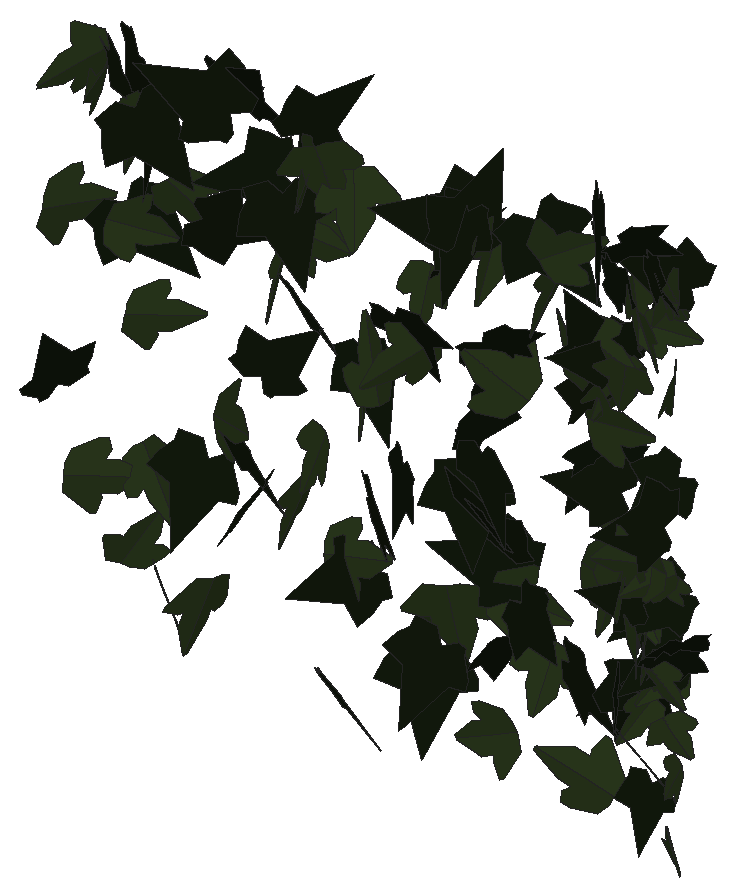
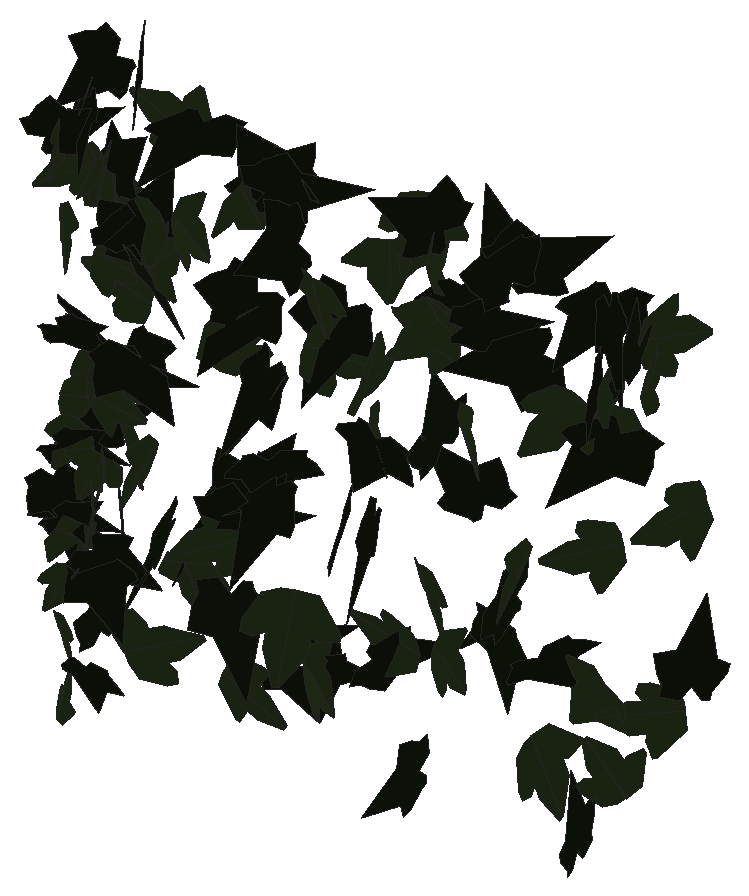
# SketchUp Ruby script. Lengths in inches.
U = 1.inch
M = Sketchup.active_model
def pt(a) = Geom::Point3d.new(a.map { |v| v * U })
def face(e, loops, mat)
  f = e.add_face(loops[0].map { |a| pt(a) })
  loops[1..].each { |l| e.add_face(l.map { |a| pt(a) }).erase! }
  f.material = f.back_material = mat if mat
  f
end
# faces: each face lists its corners as indices into pts; further lists are holes
def faces(e, pts, list, mat = nil) = list.each { |f| face(e, (f[0].is_a?(Array) ? f : [f]).map { |l| l.map { |i| pts[i] } }, mat) }
# xy, xz, yz: faces in a plane at the given z, y or x. An outline is a flat list of corners, or four numbers for a rectangle; further outlines are holes
def ring(l) = l.size == 4 ? [[l[0], l[1]], [l[2], l[1]], [l[2], l[3]], [l[0], l[3]]] : l.each_slice(2).to_a
def flat(e, list, mat, &to3) = list.each { |f| face(e, (f[0].is_a?(Array) ? f : [f]).map { |l| ring(l).map { |u, v| to3.(u, v) } }, mat) }
def xy(e, z, list, mat = nil) = flat(e, list, mat) { |x, y| [x, y, z] }
def xz(e, y, list, mat = nil) = flat(e, list, mat) { |x, z| [x, y, z] }
def yz(e, x, list, mat = nil) = flat(e, list, mat) { |y, z| [x, y, z] }
def lines(e, pts, list) = list.each { |a, b| e.add_line(pt(pts[a]), pt(pts[b])) }
# prism: a flat outline (further loops are holes) pulled along v
def prism(e, loops, v, mat = nil)
  f = face(e, loops, mat); d = Geom::Vector3d.new(v.map { |x| x * U })
  f.pushpull(f.normal.samedirection?(d) ? d.length : -d.length)
end
def box(e, o, s, mat = nil) = prism(e, [[o, [o[0] + s[0], o[1], o[2]], [o[0] + s[0], o[1] + s[1], o[2]], [o[0], o[1] + s[1], o[2]]]], [0, 0, s[2]], mat)
def at(x, y, z, deg = 0) = Geom::Transformation.translation(pt([x, y, z])) * Geom::Transformation.rotation(ORIGIN, Z_AXIS, deg.degrees)
def axes(o, x, y, z) = Geom::Transformation.new([*x, 0, *y, 0, *z, 0, *pt(o).to_a, 1])
def part(name) = M.definitions.add(name)
# library, detail: a bought-in or finely detailed component or shape, given as its bounding box
def library(name, o, s) = part(name).tap { |d| box(d.entities, o, s) }
def detail(e, o, s) = box(e.add_group.entities, o, s)
def put(e, d, t, mat = nil) = e.add_instance(d, t).tap { |i| i.material = mat if mat }
def group(e, t, mat = nil) = e.add_group.tap { |g| g.transformation = t; g.material = mat if mat }.entities
root = M.entities
M.materials.add("efeu1").color = [18, 25, 13]
M.materials.add("efeu2").color = [43, 57, 29]
c1 = part("ivyleaf_10")
p = [[0,0.5,-0.03],[-0.0625,2.02,-0.43],[-0.19,2.01,-0.46],[-0.54,1.05,-0.29],[-0.52,0.625,-0.18],[-0.83,0.76,-0.28],
  [-1.16,0.64,-0.33],[-1.15,0.33,-0.24],[-0.77,-0.39,0.02],[-0.3,-0.51,0.16],[0.04,-0.48,0.23],[-0.02,2.01,-0.4375],
  [-0.06,2.01,-0.43],[0.04,-0.49,0.23],[0.67,-0.49,0.14],[1.38,0.36,-0.2],[1.375,0.51,-0.24],[0.81,0.65,-0.19],
  [0.62,0.59,-0.15],[0.6,1.09,-0.28],[0.5,1.23,-0.31]]
faces(c1.entities,p,[[0,1,2,3,4,5,6,7,8,9,10],[11,12,0,13,14,15,16,17,18,19,20]],"efeu2")
c2 = part("ivyleaf_9")
p = [[1.54,2.16,1.25],[1.36,2.04,1.19],[-0.21,0.99,0.68],[-0.71,1.11,0.82],[-0.85,0.86,0.67],[-0.8,0.17,0.21],
  [-0.9,-0.01,0.1],[-0.67,-0.16,-0.02],[-0.08,-0.08,-0.05],[-0.03,-0.6,-0.4],[0.65,-0.88,-0.66],[0.83,-0.6,-0.49],
  [1.29,-0.42,-0.43],[1.8125,-0.07,-0.26],[1.21,0.44,0.15]]
faces(c2.entities,p,[[0,1,2,3,4,5,6,7,8,9,10,11,12,13,14]],"efeu1")
put(root,c1,axes([566.49,126.68,186.625],[-0.10386,-1.14603,0.30004],[-0.01934,-0.29951,-1.1507],[1.1845,-0.10538,0.00753]))
put(root,c2,axes([577.23,126.6875,204.34],[-0.88932,-0.20314,-0.54791],[0.53576,0.11491,-0.9122],[0.23331,-1.03821,0.00624]))
put(root,c2,axes([584.02,125.99,189.29],[-0.02279,0.04016,-0.77086],[-0.73825,0.2241,0.0335],[0.22544,0.73792,0.03178]))
put(root,c1,axes([574.99,127.1,198.43],[-0.15736,-0.47217,1.00902],[-0.32096,-0.95661,-0.4977],[1.06679,-0.35746,-0.0009]))
put(root,c1,axes([584.31,126.42,194.1],[-0.19193,-0.01617,0.84219],[-0.82302,-0.18038,-0.19102],[0.17941,-0.84474,0.02467]))
put(root,c1,axes([584.07,126.39,201.02],[-0.76472,-0.25066,0.21201],[-0.20317,-0.06083,-0.80474],[0.25788,-0.79123,-0.0053]))
put(root,c1,axes([573.87,126.07,197.08],[-0.15188,1.1664,-0.31602],[-0.09155,0.30649,1.17521],[1.20498,0.1703,0.04945]))
put(root,c2,axes([569.73,126.59,202.38],[-0.22189,-0.87568,-0.56529],[0.1674,0.54052,-0.903],[1.02876,-0.27682,0.02501]))
put(root,c2,axes([575.72,127.13,187.55],[-0.47267,-0.91093,0.18622],[-0.07425,-0.17125,-1.02618],[0.9268,-0.4783,0.01276]))
put(root,c2,axes([564.03,126.18,203.76],[-0.0359,-0.626,-0.94105],[0.10369,0.93573,-0.62642],[1.12548,-0.10618,0.0277]))
put(root,c2,axes([584.17,126.98,192.25],[-0.15493,-0.08078,0.76958],[-0.691,-0.33882,-0.17467],[0.34829,-0.70814,-0.00422]))
put(root,c2,axes([582.35,127.13,206.23],[-0.06176,0.05022,-1.17516],[1.08847,-0.44358,-0.07616],[-0.44581,-1.08997,-0.02315]))
put(root,c1,axes([570.23,127.3,203.44],[0.0958,-0.09945,1.12868],[0.73135,-0.85972,-0.13782],[0.86541,0.73755,-0.00847]))
put(root,c2,axes([577.57,127.07,195.3],[0.42299,-1.01626,0.30323],[0.11788,-0.27939,-1.10077],[1.05396,0.4391,0.00142]))
put(root,c1,axes([584.6875,125.98,191.03],[0.03021,0.16335,-0.91459],[-0.37824,0.83796,0.13717],[0.84858,0.36769,0.0937]))
put(root,c2,axes([585.4,126.54,195.71],[-0.85724,0.43641,0.47899],[-0.4303,0.21054,-0.96191],[-0.4845,-0.95915,0.0068]))
put(root,c1,axes([571.34,126.46,204.54],[-0.88843,-0.62522,-0.23962],[0.19553,0.13851,-1.08637],[0.64037,-0.90969,-0.00073]))
put(root,c1,axes([561.72,126.18,189.55],[-0.09088,-0.06928,-1.08662],[0.97152,0.48718,-0.11231],[0.49163,-0.97553,0.02108]))
put(root,c1,axes([580.88,126.53,204.12],[-0.5187,-0.29308,0.90553],[0.78598,0.4497,0.59576],[-0.53677,0.9417,-0.00268]))
put(root,c1,axes([583.24,126.83,192.9375],[0.89899,-0.72337,-0.15791],[-0.11414,0.11002,-1.1538],[0.73156,0.90609,0.01403]))
put(root,c1,axes([584.96,127.24,193.36],[-0.06928,-0.1803,0.7382],[-0.27367,-0.6856,-0.19314],[0.70891,-0.28229,-0.00241]))
put(root,c1,axes([582.45,126.99,184.88],[0.44782,0.28826,1.04519],[-0.90957,-0.51558,0.53191],[0.59009,-1.01348,0.02669]))
put(root,c2,axes([581.8,126.42,189.33],[0.84066,-0.43945,-0.68809],[-0.57575,0.38117,-0.94685],[0.57888,1.0173,0.05754]))
put(root,c2,axes([579.74,126.48,190.81],[0.48369,-0.56875,-0.69273],[-0.40981,0.55973,-0.7457],[0.79713,0.63288,0.03698]))
put(root,c2,axes([574.61,126.39,199.71],[1.04054,0.33777,-0.35353],[-0.33606,-0.10976,-1.09399],[-0.35516,1.09347,-0.0006]))
put(root,c2,axes([566.88,126.21,200.75],[0.27784,0.29984,-0.99452],[0.37322,0.93192,0.38524],[0.96937,-0.44474,0.13673]))
put(root,c2,axes([577.02,127.21,203.55],[-0.5547,-0.00509,1.03255],[-1.03063,-0.06895,-0.55401],[0.06314,-1.17008,0.02816]))
put(root,c2,axes([573.43,126.46,192.51],[0.71617,-0.23395,-0.85494],[-0.81427,0.26057,-0.75341],[0.35017,1.0844,-0.00341]))
put(root,c2,axes([566.87,127.2,204.31],[-0.15158,0.0607,1.14922],[-1.14997,-0.05262,-0.1489],[0.04431,-1.15798,0.06701]))
put(root,c1,axes([563.28,126.3,199.25],[0.23571,0.2544,0.92554],[0.37873,0.85106,-0.33038],[-0.88199,0.43344,0.10549]))
put(root,c1,axes([560.88,127.77,204.1],[0.01425,-0.18041,1.09376],[-0.01951,-1.09372,-0.18015],[1.10837,-0.01693,-0.01723]))
put(root,c2,axes([565.72,127.58,190.76],[-0.48135,-0.97775,0.09544],[-0.04148,-0.08596,-1.08982],[0.98153,-0.48313,0.00075]))
put(root,c2,axes([559.82,127.29,191.79],[0.48073,0.43756,0.72981],[-0.52722,-0.50478,0.64993],[0.66792,-0.71339,-0.01225]))
put(root,c1,axes([584.92,126.74,193.9],[0.07508,-0.0076,-0.93912],[-0.83617,0.42839,-0.07032],[0.42758,0.83909,0.0274]))
put(root,c2,axes([577.25,126.6,203.57],[-0.59382,-0.23025,0.85214],[0.79058,0.31805,0.63686],[-0.3926,0.98874,-0.00642]))
put(root,c1,axes([572.53,127.43,196.42],[0.60031,-0.63921,0.55004],[0.41804,-0.3608,-0.87554],[0.73238,0.72989,0.0489]))
put(root,c2,axes([568.25,126.44,190.3125],[-0.23739,0.92759,0.36764],[-0.08959,0.35656,-0.95748],[-0.99376,-0.25373,-0.0015]))
put(root,c1,axes([563.15,126.9,186.74],[-0.44242,-0.72861,0.42578],[0.2236,0.36235,0.85241],[-0.81374,0.49571,0.00274]))
put(root,c2,axes([575.29,127.45,186.9375],[-0.55523,-0.93141,-0.33338],[0.16387,0.29043,-1.08432],[0.97561,-0.57886,-0.0076]))
put(root,c2,axes([583.91,126.5,205.73],[0.56615,0.544,0.36343],[0.26453,0.24924,-0.78515],[-0.59837,0.62489,-0.00323]))
put(root,c1,axes([580.2,127.22,188.76],[1.04105,0.05624,-0.12869],[-0.1288,-0.00155,-1.04256],[-0.05601,1.04897,0.00536]))
put(root,c1,axes([569.82,127.32,200.91],[-0.02759,-0.06474,-1.11764],[1.06053,-0.35961,-0.00535],[-0.35859,-1.05857,0.07016]))
put(root,c2,axes([579.98,126.94,204.86],[0.06666,-0.71013,-0.93458],[0.22422,0.92655,-0.68804],[1.15215,-0.13923,0.18797]))
put(root,c2,axes([568.56,127.03,195.25],[-0.24923,0.02793,0.93591],[0.90727,-0.23219,0.24853],[0.23144,0.94028,0.03357]))
put(root,c1,axes([577.84,127.55,203.4],[0.12083,0.96582,-0.60447],[-0.13836,-0.59093,-0.97183],[-1.13095,0.17548,0.05431]))
put(root,c1,axes([563.52,127.28,190.2],[0.84985,0.03534,0.75846],[0.75622,0.06284,-0.85027],[-0.06819,1.13735,0.02341]))
put(root,c2,axes([567.11,127.2,192.31],[0.88102,-0.58861,-0.09034],[-0.06516,0.06506,-1.05941],[0.59193,0.88325,0.01784]))
put(root,c1,axes([574.96,127.39,200.87],[0.94158,-0.20378,0.04962],[0.04944,-0.00616,-0.96337],[0.20383,0.94286,0.00444]))
put(root,c1,axes([567.27,126.59,193.3],[-0.2925,0.59897,0.81223],[-0.36437,0.72593,-0.66655],[-0.94112,-0.46721,0.00562]))
put(root,c2,axes([578.6,127.52,191.2],[-0.4169,0.07426,0.97496],[-0.97636,0.02562,-0.41945],[-0.0528,-1.06005,0.05816]))
put(root,c1,axes([578.3,127.1875,185.28],[0.46895,-0.09222,-0.95319],[-0.91224,0.27989,-0.47589],[0.29136,1.02477,0.04419]))
put(root,c1,axes([582.24,127.28,198.07],[-0.23863,-0.13511,1.13339],[1.12034,0.19375,0.25898],[-0.21832,1.14192,0.09016]))
put(root,c2,axes([576.72,127.58,194.01],[-0.43773,-0.85574,-0.42712],[0.20383,0.37547,-0.96115],[0.93444,-0.48277,0.00957]))
put(root,c2,axes([571.96,128.1,188.74],[0.0415,-0.51476,-0.88394],[0.04015,-0.88316,0.5162],[-1.02211,-0.05559,-0.01562]))
put(root,c2,axes([563.93,127.96,184.64],[-0.02034,-0.27964,1.0367],[0.33388,-0.98714,-0.25972],[1.02053,0.31738,0.10563]))
put(root,c2,axes([577.875,127.47,191.89],[0.59384,-0.31867,0.91282],[-0.80958,0.42175,0.67391],[-0.52857,-1.004,-0.00664]))
put(root,c2,axes([571,127.24,184.625],[0.88085,-0.42555,-0.01649],[-0.01111,0.01493,-0.97822],[0.42572,0.88088,0.00861]))
put(root,c1,axes([571.96,127.39,203.3],[0.79394,0.74825,0.04289],[0.02946,0.03128,-1.09096],[-0.74889,0.79448,0.00256]))
put(root,c2,axes([584.39,127.22,204.89],[0.58435,-0.35471,-0.51488],[-0.45119,0.24864,-0.68337],[0.43284,0.73807,-0.01723]))
put(root,c2,axes([573.4375,128.1,192.97],[0.2119,-0.14882,-1.00993],[0.87625,-0.50267,0.25792],[-0.52374,-0.90121,0.02292]))
put(root,c1,axes([583.91,127.47,202.33],[-0.5649,0.50785,-0.26119],[0.19244,-0.17661,-0.75962],[-0.53768,-0.59677,0.00254]))
put(root,c2,axes([563,127.05,199.51],[-0.07176,-0.43035,-1.09772],[0.22216,1.07512,-0.43602],[1.15795,-0.23294,0.01562]))
put(root,c2,axes([569.32,128.1,197.61],[0.8455,-0.26924,-0.63782],[0.59204,-0.24068,0.88642],[-0.35887,-1.03139,-0.04035]))
put(root,c2,axes([582.64,128.12,200.06],[-0.25807,-0.15753,0.90194],[-0.78906,-0.43706,-0.30211],[0.46443,-0.83011,-0.0121]))
put(root,c1,axes([571.23,127.65,189.26],[0.20078,-0.18276,-1.06134],[1.03502,-0.26562,0.24154],[-0.29763,-1.04699,0.12399]))
put(root,c1,axes([578.16,127.97,197.625],[0.29034,0.83928,0.77489],[-0.24124,-0.73644,0.88803],[1.11653,-0.37736,-0.00964]))
put(root,c1,axes([583.75,127.92,187.88],[0.22696,0.44742,-0.58137],[-0.28949,-0.50455,-0.50131],[-0.67407,0.36733,0.01955]))
put(root,c2,axes([583.21,128.01,185.9],[0.74879,-0.34488,-0.24894],[0.22501,-0.10653,0.82439],[-0.36094,-0.78186,-0.00252]))
put(root,c2,axes([582,127.78,200.31],[0.53666,0.19001,0.81989],[-0.8304,-0.03868,0.5525],[0.13695,-0.97914,0.13728]))
put(root,c2,axes([568.26,128.13,202.14],[-0.51777,-0.25859,0.76669],[-0.70832,-0.29511,-0.57789],[0.3911,-0.87682,-0.03161]))
put(root,c1,axes([581.625,127.59,201],[-0.46308,0.02011,-0.88147],[0.86949,-0.15471,-0.46032],[-0.14623,-0.98362,0.05438]))
put(root,c2,axes([582.6,127.78,195.48],[-0.56566,0.16615,0.72328],[-0.71854,0.10477,-0.58602],[-0.18556,-0.91221,0.06443]))
put(root,c1,axes([570.04,127.45,201.47],[-0.72056,-0.22656,-0.62415],[0.58981,0.20465,-0.7552],[0.30498,-0.93106,-0.01412]))
put(root,c1,axes([584.3125,127.68,189.42],[-0.55213,0.03677,-0.46637],[0.45942,-0.0935,-0.55127],[-0.08826,-0.71667,0.04799]))
put(root,c1,axes([562.37,128.41,202.02],[-0.00286,-0.46987,0.95246],[0.57081,-0.80388,-0.39486],[0.89562,0.51084,0.2547]))
put(root,c1,axes([582.74,128.31,199.63],[-0.04285,-0.56802,0.7349],[-0.03248,-0.73431,-0.56946],[0.92826,-0.05192,0.014]))
put(root,c2,axes([583.34,128.11,188.66],[0.00576,0.02618,-0.85804],[-0.31482,-0.79821,-0.02647],[-0.79862,0.31484,0.00424]))
put(root,c1,axes([578.47,127.24,190.39],[0.29311,0.17426,1.04511],[0.75367,0.72788,-0.33274],[-0.74472,0.80521,0.07461]))
put(root,c2,axes([584.61,128.29,192.22],[-0.71868,-0.45227,0.35496],[-0.30452,-0.18254,-0.84912],[0.48767,-0.7805,-0.00711]))
put(root,c1,axes([583.11,128.1,191.49],[-0.26207,0.52515,-0.66833],[0.28357,-0.60528,-0.58681],[-0.80127,-0.38597,0.01091]))
put(root,c2,axes([576.6875,127.39,192.95],[1.10088,0.06019,-0.50232],[-0.50146,-0.02957,-1.10253],[-0.06703,1.20971,-0.00195]))
put(root,c2,axes([570.03,127.21,204.69],[-0.02933,-0.01886,0.99555],[0.87599,0.47306,0.03476],[-0.47342,0.87647,0.00266]))
put(root,c1,axes([583.41,128.24,190.2],[-0.19422,0.40528,-0.73926],[0.2349,-0.70256,-0.44688],[-0.80967,-0.30105,0.04768]))
put(root,c2,axes([577.65,127.16,199.54],[0.74219,0.74828,0.16011],[0.1131,0.11333,-1.05393],[-0.75681,0.75076,-0.00048]))
put(root,c2,axes([566.51,128.12,204.53],[1.08278,-0.09705,-0.23007],[0.23712,0.07867,1.08275],[-0.07828,-1.10415,0.09737]))
put(root,c1,axes([574.34,128.34,187.51],[0.42459,-0.87307,0.54689],[0.25617,-0.48346,-0.9707],[0.99786,0.49561,0.0165]))
put(root,c2,axes([584.61,128.26,196.47],[-0.76058,-0.39214,0.11602],[-0.10531,-0.04892,-0.85571],[0.39516,-0.76782,-0.00474]))
put(root,c2,axes([581.83,127.54,199.21],[-0.55414,0.68761,0.39468],[-0.266,0.29237,-0.88285],[-0.74688,-0.6143,0.0216]))
put(root,c1,axes([581.21,127.53,199.65],[-0.52316,0.42478,-0.76592],[-0.57917,0.50145,0.67371],[0.65699,0.78031,-0.016]))
put(root,c1,axes([563.26,127.33,195.53],[-0.18017,-0.09049,-1.02991],[0.82912,0.61188,-0.19881],[0.61762,-0.84781,-0.03356]))
put(root,c2,axes([584.11,127.58,204.54],[0.46775,-0.0122,-0.6866],[-0.68026,0.10535,-0.4653],[0.09389,0.82408,0.04932]))
put(root,c2,axes([584.83,127.76,190.14],[0.33183,0.55997,-0.39745],[-0.1973,-0.34506,-0.65088],[-0.65772,0.38602,-0.00527]))
put(root,c2,axes([577.21,127.1,196.89],[0.05699,0.05625,-1.16507],[-0.75506,0.89087,0.00608],[0.88906,0.75298,0.07984]))
put(root,c1,axes([575.6875,127.82,189.1],[-1.10513,-0.5953,-0.11681],[0.10618,0.04919,-1.25525],[0.59729,-1.11019,0.00702]))
put(root,c2,axes([572,128.07,196.66],[-0.51683,-0.34664,-0.82599],[0.69025,0.45369,-0.62229],[0.57094,-0.86228,0.00463]))
put(root,c1,axes([579.45,128.52,202.07],[0.30252,-0.79694,0.60526],[0.2005,-0.57123,-0.85234],[0.98044,0.36271,-0.01245]))
put(root,c1,axes([560.49,128.625,202.85],[-0.10815,0.08717,0.99849],[0.6127,-0.78903,0.13525],[0.7932,0.62137,0.03167]))
put(root,c1,axes([583.06,127.92,194.19],[0.1152,0.09453,-0.81765],[-0.79468,0.22784,-0.08562],[0.21441,0.79367,0.12196]))
put(root,c1,axes([584.76,128.04,182.44],[-0.548,0.39423,0.0178],[0.01155,-0.01442,0.67505],[0.39446,0.5481,0.00495]))
put(root,c2,axes([561.28,128.79,203.14],[-0.15778,-0.37145,1.00974],[0.23758,-1.00738,-0.33346],[1.04934,0.17223,0.22733]))
put(root,c1,axes([583.3,127.92,191.77],[0.62551,0.33108,0.39964],[0.33799,0.21506,-0.70718],[-0.39381,0.71044,0.02783]))
put(root,c2,axes([585.08,127.99,190.62],[-0.07987,0.67637,-0.39898],[-0.13324,-0.4069,-0.66312],[-0.7739,0.00025,0.15535]))
put(root,c2,axes([578.16,127.6875,188.6],[-0.10074,1.12246,-0.18283],[0.00633,-0.18299,-1.12693],[-1.13724,-0.10045,0.00992]))
put(root,c2,axes([581.9,128.26,196.56],[0.10924,0.57812,-0.81132],[-0.1217,-0.80233,-0.58809],[-0.98876,0.16262,-0.01725]))
put(root,c1,axes([584.74,127.93,200.24],[0.29779,-0.73847,-0.31247],[-0.05059,0.31535,-0.79351],[0.80026,0.29473,0.06611]))
put(root,c2,axes([562.72,128.64,202.16],[-0.06717,0.05527,-1.07583],[0.9518,-0.50179,-0.0852],[-0.50453,-0.95401,-0.01751]))
put(root,c1,axes([584.32,127.97,192.67],[-0.69466,-0.0574,-0.24092],[0.24044,0.01573,-0.69702],[0.05938,-0.73509,0.0039]))
put(root,c1,axes([564.45,127.83,200.33],[-0.80578,-0.27829,-0.64718],[0.60561,0.2287,-0.85236],[0.3599,-1.00789,-0.01471]))
put(root,c2,axes([584.34,128.63,189.81],[-0.59669,-0.46632,0.34208],[-0.27235,-0.20703,-0.75728],[0.51019,-0.6559,-0.00418]))
put(root,c2,axes([583.27,128.07,188.02],[0.31724,0.47444,-0.6402],[-0.38437,-0.5125,-0.57026],[-0.69801,0.49784,0.02306]))
put(root,c1,axes([584.28,128.53,189.3],[0.28027,0.45208,-0.66383],[-0.35198,-0.56284,-0.5319],[-0.72191,0.44993,0.00162]))
put(root,c2,axes([582.61,127.94,202.63],[0.19395,-0.29838,0.81868],[-0.43054,0.69636,0.3558],[-0.75756,-0.47215,0.00738]))
put(root,c1,axes([581.74,127.5,192.48],[-0.17852,0.61126,0.71456],[-0.24238,0.67284,-0.63611],[-0.90856,-0.29959,0.0293]))
put(root,c1,axes([568.12,128.4,198.61],[0.6212,-0.77185,0.22562],[0.15023,-0.16868,-0.99072],[0.78999,0.63901,0.01099]))
put(root,c1,axes([584.2,127.66,202.16],[0.19462,0.14726,0.77938],[0.42695,0.65687,-0.23073],[-0.66846,0.46242,0.07954]))
put(root,c1,axes([584.66,127.86,203.65],[0.05939,-0.749,-0.45356],[0.17981,0.45534,-0.7284],[0.85696,-0.04363,0.18427]))
put(root,c1,axes([584.5,128.07,187.38],[-0.46474,-0.4114,-0.32887],[0.34576,0.09255,-0.60438],[0.39731,-0.56176,0.14127]))
put(root,c1,axes([583.03,128.22,202.92],[-0.16993,0.91344,-0.21342],[0.0412,-0.20942,-0.92911],[-0.93714,-0.17484,-0.00215]))
put(root,c1,axes([569.83,128.26,192.53],[0.81841,-0.56988,-0.2026],[-0.15499,0.1319,-0.99709],[0.58462,0.83273,0.01929]))
put(root,c1,axes([568.8,128.68,190.25],[0.21101,-0.79797,0.49323],[0.15281,-0.46957,-0.82506],[0.92557,0.25944,0.02377]))
put(root,c2,axes([575.86,127.33,202.12],[0.25502,0.48483,0.93654],[0.36799,0.86207,-0.54647],[-0.98831,0.44608,0.03818]))
put(root,c1,axes([559.64,127.45,198.25],[-0.14679,-0.22822,-1.12616],[0.55315,0.98107,-0.27092],[1.00715,-0.57209,-0.01535]))
put(root,c2,axes([583.41,128.48,184.54],[-0.61204,-0.28799,-0.40135],[0.3613,0.17481,-0.6764],[0.33687,-0.71072,-0.00374]))
put(root,c1,axes([584.6875,128.2,185.65],[0.50613,-0.41752,-0.28536],[-0.20127,0.20407,-0.65557],[0.46394,0.54402,0.02691]))
put(root,c2,axes([584.84,128.6,203.51],[-0.14529,0.00639,0.88965],[-0.88112,-0.1257,-0.143],[0.12304,-0.89263,0.02651]))
put(root,c2,axes([562.62,127.93,204.54],[0.40444,0.00846,-1.01913],[-1.01916,0.00164,-0.40444],[-0.0016,1.09644,0.00847]))
